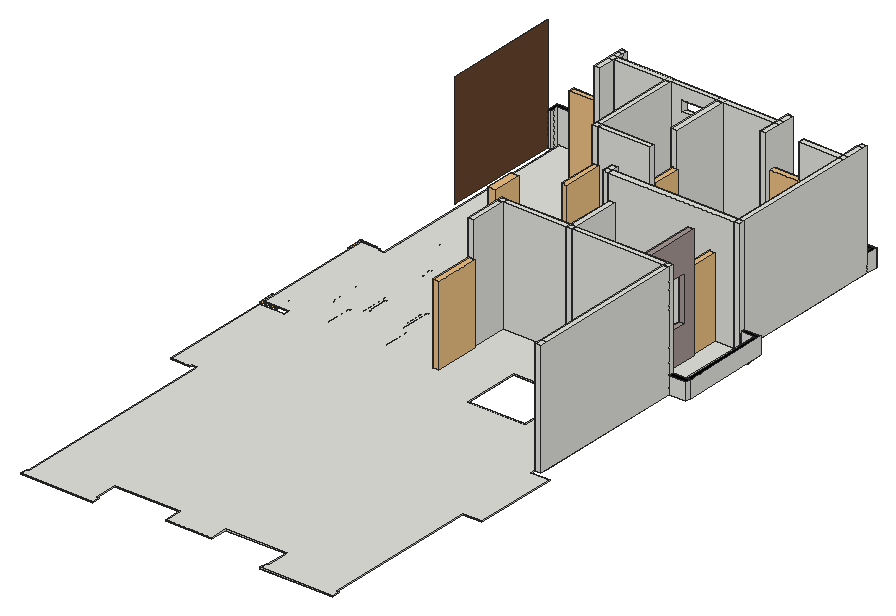
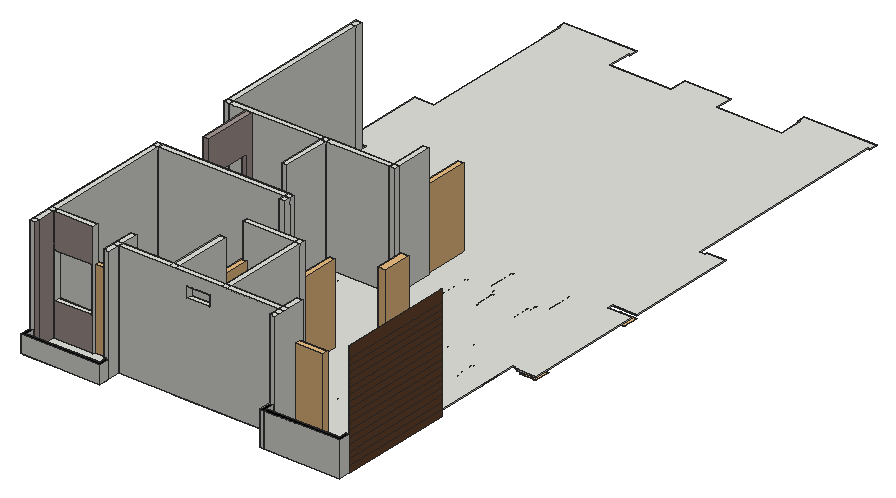
# SketchUp Ruby script. Lengths in inches.
U = 1.inch
M = Sketchup.active_model
def pt(a) = Geom::Point3d.new(a.map { |v| v * U })
def face(e, loops, mat)
  f = e.add_face(loops[0].map { |a| pt(a) })
  loops[1..].each { |l| e.add_face(l.map { |a| pt(a) }).erase! }
  f.material = f.back_material = mat if mat
  f
end
# faces: each face lists its corners as indices into pts; further lists are holes
def faces(e, pts, list, mat = nil) = list.each { |f| face(e, (f[0].is_a?(Array) ? f : [f]).map { |l| l.map { |i| pts[i] } }, mat) }
# xy, xz, yz: faces in a plane at the given z, y or x. An outline is a flat list of corners, or four numbers for a rectangle; further outlines are holes
def ring(l) = l.size == 4 ? [[l[0], l[1]], [l[2], l[1]], [l[2], l[3]], [l[0], l[3]]] : l.each_slice(2).to_a
def flat(e, list, mat, &to3) = list.each { |f| face(e, (f[0].is_a?(Array) ? f : [f]).map { |l| ring(l).map { |u, v| to3.(u, v) } }, mat) }
def xy(e, z, list, mat = nil) = flat(e, list, mat) { |x, y| [x, y, z] }
def xz(e, y, list, mat = nil) = flat(e, list, mat) { |x, z| [x, y, z] }
def yz(e, x, list, mat = nil) = flat(e, list, mat) { |y, z| [x, y, z] }
def lines(e, pts, list) = list.each { |a, b| e.add_line(pt(pts[a]), pt(pts[b])) }
# prism: a flat outline (further loops are holes) pulled along v
def prism(e, loops, v, mat = nil)
  f = face(e, loops, mat); d = Geom::Vector3d.new(v.map { |x| x * U })
  f.pushpull(f.normal.samedirection?(d) ? d.length : -d.length)
end
def box(e, o, s, mat = nil) = prism(e, [[o, [o[0] + s[0], o[1], o[2]], [o[0] + s[0], o[1] + s[1], o[2]], [o[0], o[1] + s[1], o[2]]]], [0, 0, s[2]], mat)
def at(x, y, z, deg = 0) = Geom::Transformation.translation(pt([x, y, z])) * Geom::Transformation.rotation(ORIGIN, Z_AXIS, deg.degrees)
def axes(o, x, y, z) = Geom::Transformation.new([*x, 0, *y, 0, *z, 0, *pt(o).to_a, 1])
def part(name) = M.definitions.add(name)
# library, detail: a bought-in or finely detailed component or shape, given as its bounding box
def library(name, o, s) = part(name).tap { |d| box(d.entities, o, s) }
def detail(e, o, s) = box(e.add_group.entities, o, s)
def put(e, d, t, mat = nil) = e.add_instance(d, t).tap { |i| i.material = mat if mat }
def group(e, t, mat = nil) = e.add_group.tap { |g| g.transformation = t; g.material = mat if mat }.entities
root = M.entities
M.materials.add("M09_Shadow_Night").color = [0, 0, 0]
M.materials.add("Marble_06_1K").color = [165, 150, 147]
M.materials.add("Wood_Veneer_15_1K").color = [103, 69, 45]
c1 = part("Group\#84")
xy(c1.entities,0,[[[-2,-32,-2,-24,0.04,-24,0.04,0,0,0,0,198,-6,198,-6,196,-25.9,196,-25.9,312.57,0,312.57,0,318.21,-25.9,318.21,-25.9,446,-6,446,-6,444,0,444,0,675.78,72,673.93,76,673.93,76,665.93,74,665.93,74,636,252.4,636,252.4,673.93,328.4,673.93,328.4,636,324.4,636,324.4,498.14,330.4,498.14,330.4,499.84,344.35,499.84,344.35,411,324.4,411,324.4,231,344.35,231,344.35,142,324.4,142,324.4,0,324.58,0,324.58,-24,326.4,-24,326.4,-32,250.4,-32,250.4,-24,252.4,-24,252.4,0,188.4,0,188.4,-18,140,-18,140,0,72,0,72,-24,74,-24,74,-32],[210.4,291,270.4,351]]])
xy(c1.entities,1,[[[-2,-32,74,-32,74,-24,72,-24,72,0,140,0,140,-18,188.4,-18,188.4,0,252.4,0,252.4,-24,250.4,-24,250.4,-32,326.4,-32,326.4,-24,324.58,-24,324.58,0,324.4,0,324.4,142,344.35,142,344.35,231,324.4,231,324.4,411,344.35,411,344.35,499.84,330.4,499.84,330.4,498.14,324.4,498.14,324.4,636,328.4,636,328.4,673.93,252.4,673.93,252.4,636,74,636,74,665.93,76,665.93,76,673.93,72,673.93,0,675.78,0,444,-6,444,-6,446,-25.9,446,-25.9,318.21,0,318.21,0,312.57,-25.9,312.57,-25.9,196,-6,196,-6,198,0,198,0,0,0.04,0,0.04,-24,-2,-24],[210.4,291,270.4,351]]])
xz(c1.entities,-32,[[-2,0,74,1],[250.4,0,326.4,1]])
xz(c1.entities,-24,[[-2,0,0.04,1],[72,0,74,1],[250.4,0,252.4,1],[324.58,0,326.4,1]])
xz(c1.entities,-18,[[140,0,188.4,1]])
xz(c1.entities,0,[[0,0,0.04,1],[72,0,140,1],[188.4,0,252.4,1],[324.4,0,324.58,1]])
xz(c1.entities,142,[[324.4,0,344.35,1]])
xz(c1.entities,196,[[-25.9,0,-6,1]])
xz(c1.entities,198,[[-6,0,0,1]])
xz(c1.entities,231,[[324.4,0,344.35,1]])
xz(c1.entities,291,[[210.4,0,270.4,1]])
xz(c1.entities,312.57,[[-25.9,0,0,1]])
xz(c1.entities,318.21,[[-25.9,0,0,1]])
xz(c1.entities,351,[[210.4,0,270.4,1]])
xz(c1.entities,411,[[324.4,0,344.35,1]])
xz(c1.entities,444,[[-6,0,0,1]])
xz(c1.entities,446,[[-25.9,0,-6,1]])
xz(c1.entities,498.14,[[324.4,0,330.4,1]])
xz(c1.entities,499.84,[[330.4,0,344.35,1]])
xz(c1.entities,636,[[74,0,252.4,1],[324.4,0,328.4,1]])
xz(c1.entities,665.93,[[74,0,76,1]])
xz(c1.entities,673.93,[[72,0,76,1],[252.4,0,328.4,1]])
yz(c1.entities,-25.9,[[196,0,312.57,1],[318.21,0,446,1]])
yz(c1.entities,-6,[[196,0,198,1],[444,0,446,1]])
yz(c1.entities,-2,[[-32,0,-24,1]])
yz(c1.entities,0,[[0,0,198,1],[312.57,0,318.21,1],[444,0,636,1],[636,0,637.85,1],[637.85,0,675.78,1]])
yz(c1.entities,0.04,[[-24,0,0,1]])
yz(c1.entities,72,[[-24,0,0,1]])
yz(c1.entities,74,[[-32,0,-24,1],[636,0,665.93,1]])
yz(c1.entities,76,[[665.93,0,673.93,1]])
yz(c1.entities,140,[[-18,0,0,1]])
yz(c1.entities,188.4,[[-18,0,0,1]])
yz(c1.entities,210.4,[[291,0,351,1]])
yz(c1.entities,250.4,[[-32,0,-24,1]])
yz(c1.entities,252.4,[[-24,0,0,1],[636,0,673.93,1]])
yz(c1.entities,270.4,[[291,0,351,1]])
yz(c1.entities,324.4,[[0,0,142,1],[231,0,411,1],[498.14,0,636,1]])
yz(c1.entities,324.58,[[-24,0,0,1]])
yz(c1.entities,326.4,[[-32,0,-24,1]])
yz(c1.entities,328.4,[[636,0,673.93,1]])
yz(c1.entities,330.4,[[498.14,0,499.84,1]])
yz(c1.entities,344.35,[[142,0,231,1],[411,0,499.84,1]])
# 3 loose lines left out
p = [[77.67,648,0],[77.67,636,1],[246.4,636,1],[246.4,648,0],[72,673.93,0],[0,675.78,0],
  [0,675.78,1],[72,673.93,1]]
faces(c1.entities,p,[[0,1,2,3],[4,5,6,7]])
c2 = library("TREE-26",[-60.96,-72.91,0],[121.92,134.74,0.01])
c3 = library("HYHHYHYHYHYHY",[-2.09,-4.54,0],[4.18,9.08,0.01])
c4 = library("Group\#51",[0,0,0],[6.9375,42,86.5])
c5 = part("feeeeeeeeee")
p = [[-2.68,3.51,0],[-2.68,3.16,0],[-2.92,3.16,0],[-2.92,3.07,0],[-3.56,3.07,0],[-3.56,3.51,0],
  [-2.68,-3.51,0],[-2.68,-3.16,0],[-2.92,-3.16,0],[-2.92,-3.07,0],[-3.56,-3.07,0],[-3.56,-3.51,0],
  [3.56,3.16,0],[-2.68,2.93,0],[3.56,2.93,0],[-2.48,-3.13,0],[-2.04,-3.07,0],[-1.61,-2.98,0],
  [-1.1875,-2.86,0],[-0.77,-2.72,0],[-0.36,-2.55,0],[0.03,-2.35,0],[0.41,-2.13,0],[0.78,-1.88,0],
  [1.125,-1.62,0],[1.46,-1.32,0],[1.77,-1.01,0],[2.06,-0.68,0],[2.33,-0.33,0],[2.57,0.03,0],
  [2.79,0.42,0],[2.99,0.81,0],[3.16,1.22,0],[3.3,1.63,0],[3.41,2.06,0],[3.5,2.49,0]]
lines(c5.entities,p,[[0,1],[1,2],[2,3],[3,4],[4,5],[5,0],[6,7],[7,8],[8,9],[9,10],[10,11],[11,6],
  [1,12],[13,14],[1,13],[12,14],[8,15],[15,16],[16,17],[17,18],[18,19],[19,20],[20,21],[21,22],
  [22,23],[23,24],[24,25],[25,26],[26,27],[27,28],[28,29],[29,30],[30,31],[31,32],[32,33],[33,34],
  [34,35],[35,14]])
c6 = part("Group\#12")
xy(c6.entities,0,[[0,0,6,7.18],[0,7.18,6,168],[-174.4,129.21,-168.4,168],[-174.4,168,-168.4,174],[-168.4,168,-102,174],
  [-102,168,-96,174],[-96,168,0,174],[0,168,6,174],[6,168,24,174],[-102,174,-96,225]])
xy(c6.entities,18,[[6,168,24,174]],"M09_Shadow_Night")
xy(c6.entities,120,[[0,0,6,7.18],[0,7.18,6,168],[-174.4,129.21,-168.4,168],[-174.4,168,-168.4,174],[-168.4,168,-102,174],
  [-102,168,-96,174],[-96,168,0,174],[0,168,6,174],[-102,174,-96,225]])
xz(c6.entities,0,[[0,0,6,120]])
xz(c6.entities,129.21,[[-174.4,0,-168.4,120]])
xz(c6.entities,168,[[-174.4,0,-168.4,120],[-168.4,0,-102,120],[-102,0,-96,120],[-96,0,0,120],[0,0,6,120],
  [6,0,24,18]])
xz(c6.entities,174,[[-174.4,0,-168.4,120],[-168.4,0,-102,120],[-102,0,-96,120],[-96,0,0,120],[0,0,6,120],
  [6,0,24,18]])
xz(c6.entities,225,[[-102,0,-96,120]])
yz(c6.entities,-174.4,[[129.21,0,168,120],[168,0,174,120]])
yz(c6.entities,-168.4,[[129.21,0,168,120],[168,0,174,120]])
yz(c6.entities,-102,[[168,0,174,120],[174,0,225,120]])
yz(c6.entities,-96,[[168,0,174,120],[174,0,225,120]])
yz(c6.entities,0,[[0,0,7.18,120],[7.18,0,168,120],[168,0,174,120]])
yz(c6.entities,6,[[0,0,168,120],[168,0,174,18],[168,18,174,120]])
yz(c6.entities,24,[[168,0,174,18]])
c7 = library("VVVV",[-3.39,-3.68,0],[6.78,7.36,0.01])
c8 = library("BFGFV",[-4.32,-2.51,0],[8.64,5.02,0.01])
c9 = library("burner",[-300,-225,0],[600,450,0.01])
c10 = library("lcd-01",[-577.99,-134.75,0],[1155.98,269.5,0.01])
c11 = part("Component\#5")
p = [[1166.02,522.1,0],[1167.27,522.1,0],[1183.11,522.1,0],[1183.72,522.1,0],[1165.72,517.1,0],[1167.27,517.1,0],
  [1183.11,517.1,0],[1183.72,517.1,0],[1165.72,512.1,0],[1167.27,512.1,0],[1183.11,512.1,0],[1183.72,512.1,0],
  [1165.72,507.1,0],[1167.27,507.1,0],[1183.11,507.1,0],[1183.72,507.1,0],[1165.72,502.1,0],[1167.27,502.1,0],
  [1183.11,502.1,0],[1183.72,502.1,0],[1165.72,497.1,0],[1167.27,497.1,0],[1183.11,497.1,0],[1183.72,497.1,0],
  [1165.72,492.1,0],[1183.72,492.1,0],[1165.72,487.1,0],[1183.72,487.1,0],[1111.72,482.1,0],[1128.65,482.1,0],
  [1150.05,482.1,0],[1183.72,482.1,0],[1111.72,477.1,0],[1128.65,477.1,0],[1150.05,477.1,0],[1183.72,477.1,0],
  [1111.72,472.1,0],[1128.65,472.1,0],[1150.05,472.1,0],[1173.72,472.1,0],[1117.28,469.6,0],[1112.28,474.6,0],
  [1127.28,479.6,0],[1122.28,484.6,0],[1157.28,469.6,0],[1152.28,474.6,0],[1173.72,473.16,0],[1172.28,474.6,0],
  [1167.28,479.6,0],[1162.28,484.6,0],[1183.72,483.16,0],[1182.28,484.6,0],[1177.28,489.6,0],[1172.48,494.4,0],
  [1167.27,499.61,0],[1165.72,501.16,0],[1183.72,503.16,0],[1183.11,503.77,0],[1167.27,519.61,0],[1165.77,521.11,0],
  [1183.72,523.16,0],[1182.3,524.58,0],[1118.53,469.6,0],[1113.53,474.6,0],[1128.53,479.6,0],[1123.53,484.6,0],
  [1158.53,469.6,0],[1153.53,474.6,0],[1173.72,474.41,0],[1173.53,474.6,0],[1168.53,479.6,0],[1163.53,484.6,0],
  [1183.72,484.41,0],[1183.53,484.6,0],[1178.53,489.6,0],[1173.73,494.4,0],[1167.27,500.86,0],[1165.72,502.41,0],
  [1183.72,504.41,0],[1183.53,504.6,0],[1167.27,520.86,0],[1166.02,522.11,0],[1183.72,524.41,0],[1183.55,524.58,0],
  [1119.78,469.6,0],[1114.78,474.6,0],[1128.65,480.73,0],[1124.78,484.6,0],[1159.78,469.6,0],[1154.78,474.6,0],
  [1169.78,479.6,0],[1164.78,484.6,0],[1179.78,489.6,0],[1174.98,494.4,0],[1167.27,502.11,0],[1165.72,503.66,0],
  [1167.27,522.11,0],[1166.48,522.9,0]]
lines(c11.entities,p,[[0,1],[2,3],[4,5],[6,7],[8,9],[10,11],[12,13],[14,15],[16,17],[18,19],[20,21],[22,23],
  [24,25],[26,27],[28,29],[30,31],[32,33],[34,35],[36,37],[38,39],[40,41],[42,43],[44,45],[46,47],
  [48,49],[50,51],[52,53],[54,55],[56,57],[58,59],[60,61],[62,63],[64,65],[66,67],[68,69],[70,71],
  [72,73],[74,75],[76,77],[78,79],[80,81],[82,83],[84,85],[86,87],[88,89],[90,91],[92,93],[94,95],
  [96,97]])
c12 = library("sink",[-449.92,-250,0],[899.84,500,0.01])
c13 = library("A$C72E23588",[-1177.7,-903.95,0],[2355.4,1807.9,0.01])
c14 = part("Group\#14")
xy(c14.entities,0,[[0,0,4.05,3.45],[0,3.45,4.05,88.84],[-13.95,88.84,0,93],[0,88.84,4.05,93]])
xy(c14.entities,18,[[0,0,4.05,88.84],[-13.95,88.84,0,93],[0,88.84,4.05,93]],"M09_Shadow_Night")
xz(c14.entities,0,[[0,0,4.05,18]])
xz(c14.entities,88.84,[[-13.95,0,0,18]])
xz(c14.entities,93,[[-13.95,0,4.05,18]])
yz(c14.entities,-13.95,[[88.84,0,93,18]])
yz(c14.entities,0,[[0,0,3.45,18],[3.45,0,88.84,18]])
yz(c14.entities,4.05,[[0,0,93,18]])
c15 = library("JEEW",[-211.14,-299.86,0],[422.28,599.72,0.01])
c16 = library("ghgjg",[-265.23,-341.01,0],[530.46,682.02,0.01])
c17 = part("tgr")
p = [[-2.37,-3.35,0],[-2.37,-2.82,0],[-2.73,-2.82,0],[-2.73,-2.68,0],[-3.71,-2.68,0],[-3.71,-3.35,0],
  [-2.37,3.35,0],[-2.37,2.82,0],[-2.73,2.82,0],[-2.73,2.68,0],[-3.71,2.68,0],[-3.71,3.35,0],
  [3.71,-2.82,0],[-2.37,-2.46,0],[3.71,-2.46,0],[3.7,-2.46,0],[3.63,-2.07,0],[3.53,-1.68,0],
  [3.41,-1.3,0],[3.27,-0.93,0],[3.1,-0.57,0],[2.91,-0.22,0],[2.7,0.12,0],[2.46,0.4375,0],
  [2.21,0.74,0],[1.93,1.03,0],[1.64,1.3,0],[1.33,1.55,0],[1.01,1.79,0],[0.67,1.99,0],
  [0.32,2.18,0],[-0.04,2.35,0],[-0.41,2.49,0],[-0.8,2.6,0],[-1.18,2.69,0],[-1.58,2.76,0],
  [-1.97,2.8,0]]
lines(c17.entities,p,[[0,1],[1,2],[2,3],[3,4],[4,5],[5,0],[6,7],[7,8],[8,9],[9,10],[10,11],[11,6],
  [1,12],[13,14],[1,13],[12,14],[15,16],[16,17],[17,18],[18,19],[19,20],[20,21],[21,22],[22,23],
  [23,24],[24,25],[25,26],[26,27],[27,28],[28,29],[29,30],[30,31],[31,32],[32,33],[33,34],[34,35],
  [35,36],[36,7]])
c18 = library("Group\#49",[0,0,0],[8.31,30,84])
c19 = part("EGWF")
p = [[2.59,-3.49,0],[2.59,-3.09,0],[2.85,-3.09,0],[2.85,-2.99,0],[3.58,-2.99,0],[3.58,-3.49,0],
  [2.59,3.49,0],[2.59,3.09,0],[2.85,3.09,0],[2.85,2.99,0],[3.58,2.99,0],[3.58,3.49,0],
  [-3.58,-3.09,0],[2.59,-2.82,0],[-3.58,-2.82,0],[2.2,3.07,0],[1.81,3.04,0],[1.42,2.97,0],
  [1.03,2.89,0],[0.66,2.78,0],[0.29,2.64,0],[-0.07,2.48,0],[-0.42,2.3,0],[-0.76,2.1,0],
  [-1.08,1.875,0],[-1.39,1.63,0],[-1.68,1.37,0],[-1.96,1.09,0],[-2.21,0.79,0],[-2.45,0.48,0],
  [-2.67,0.15,0],[-2.86,-0.1875,0],[-3.04,-0.54,0],[-3.1875,-0.9,0],[-3.32,-1.28,0],[-3.42,-1.66,0],
  [-3.5,-2.04,0],[-3.55,-2.43,0]]
lines(c19.entities,p,[[0,1],[1,2],[2,3],[3,4],[4,5],[5,0],[6,7],[7,8],[8,9],[9,10],[10,11],[11,6],
  [1,12],[13,14],[1,13],[12,14],[7,15],[15,16],[16,17],[17,18],[18,19],[19,20],[20,21],[21,22],
  [22,23],[23,24],[24,25],[25,26],[26,27],[27,28],[28,29],[29,30],[30,31],[31,32],[32,33],[33,34],
  [34,35],[35,36],[36,37],[37,14]])
c20 = library("double bed",[-999.9375,-1062.5,0],[1999.875,2125,0.01])
c21 = part("Group\#116")
xy(c21.entities,0,[[24,0,24.75,24.75]])
xy(c21.entities,107,[[24,0,24.75,24.75]])
xz(c21.entities,0,[[24,0,24.75,107]])
xz(c21.entities,24.75,[[24,0,24.75,107]])
yz(c21.entities,24,[[0,0,24.75,6],[0,6,24.75,12],[0,12,24.75,18],[0,18,24.75,24],[0,24,24.75,30],
  [0,30,24.75,36],[0,36,24.75,42],[0,42,24.75,48],[0,48,24.75,54],[0,54,24.75,60],
  [0,60,24.75,66],[0,66,24.75,72],[0,72,24.75,78],[0,78,24.75,84],[0,84,24.75,90],
  [0,90,24.75,96],[0,96,24.75,107]],"Wood_Veneer_15_1K")
yz(c21.entities,24.75,[[0,0,24.75,107]])
c22 = part("G5GTGTGT")
p = [[0.52,4.97,0],[0.52,-4.97,0],[0.36,-4.97,0],[0.36,4.97,0],[-0.08,-4.53,0],[-0.08,4.53,0],
  [0.33,4.97,0],[0.3,4.97,0],[0.28,4.96,0],[0.25,4.96,0],[0.22,4.95,0],[0.2,4.94,0],
  [0.17,4.93,0],[0.15,4.92,0],[0.12,4.9,0],[0.1,4.89,0],[0.08,4.87,0],[0.06,4.85,0],
  [0.04,4.83,0],[0.02,4.8125,0],[0,4.79,0],[-0.01,4.77,0],[-0.03,4.74,0],[-0.04,4.72,0],
  [-0.05,4.69,0],[-0.0625,4.67,0],[-0.07,4.64,0],[-0.08,4.61,0],[-0.08,4.59,0],[-0.08,4.56,0],
  [-0.08,-4.56,0],[-0.08,-4.59,0],[-0.08,-4.61,0],[-0.07,-4.64,0],[-0.0625,-4.67,0],[-0.05,-4.69,0],
  [-0.04,-4.72,0],[-0.03,-4.74,0],[-0.01,-4.77,0],[0,-4.79,0],[0.02,-4.8125,0],[0.04,-4.83,0],
  [0.06,-4.85,0],[0.08,-4.87,0],[0.1,-4.89,0],[0.12,-4.9,0],[0.15,-4.92,0],[0.17,-4.93,0],
  [0.2,-4.94,0],[0.22,-4.95,0],[0.25,-4.96,0],[0.28,-4.96,0],[0.3,-4.97,0],[0.33,-4.97,0],
  [-0.08,-1.38,0],[-0.52,-1.38,0],[-0.08,1.38,0],[-0.52,1.38,0]]
lines(c22.entities,p,[[0,1],[1,2],[2,3],[3,0],[4,5],[3,6],[6,7],[7,8],[8,9],[9,10],[10,11],[11,12],
  [12,13],[13,14],[14,15],[15,16],[16,17],[17,18],[18,19],[19,20],[20,21],[21,22],[22,23],[23,24],
  [24,25],[25,26],[26,27],[27,28],[28,29],[29,5],[4,30],[30,31],[31,32],[32,33],[33,34],[34,35],
  [35,36],[36,37],[37,38],[38,39],[39,40],[40,41],[41,42],[42,43],[43,44],[44,45],[45,46],[46,47],
  [47,48],[48,49],[49,50],[50,51],[51,52],[52,53],[53,2],[54,55],[56,57],[55,57]])
c23 = part("Group\#15")
xy(c23.entities,0,[[60,-108.67,66,-102.67],[66,-108.67,120.4,-102.67],[60,-102.67,66,-12.67],[114.4,-72.67,120.4,-12.67],[0,-30.67,6,-12.67],
  [174.4,-30.67,180.4,-12.67],[0,-12.67,6,-6.67],[6,-12.67,60,-6.67],[60,-12.67,66,-6.67],[66,-12.67,114.4,-6.67],
  [114.4,-12.67,120.4,-6.67],[120.4,-12.67,174.4,-6.67],[174.4,-12.67,180.4,-6.67],[0,-6.67,6,0],[174.4,-6.67,180.4,5.26],
  [0,0,6,5.26]])
xy(c23.entities,96,[[78,-12.67,102.4,-6.67]])
xy(c23.entities,108,[[78,-12.67,102.4,-6.67]])
xy(c23.entities,120,[[60,-108.67,66,-102.67],[66,-108.67,120.4,-102.67],[60,-102.67,66,-12.67],[114.4,-72.67,120.4,-12.67],[0,-30.67,6,-12.67],
  [174.4,-30.67,180.4,-12.67],[0,-12.67,6,-6.67],[6,-12.67,60,-6.67],[60,-12.67,66,-6.67],[66,-12.67,114.4,-6.67],
  [114.4,-12.67,120.4,-6.67],[120.4,-12.67,174.4,-6.67],[174.4,-12.67,180.4,-6.67],[0,-6.67,6,0],[174.4,-6.67,180.4,5.26],
  [0,0,6,5.26]])
xz(c23.entities,-108.67,[[60,0,66,120],[66,0,120.4,120]])
xz(c23.entities,-102.67,[[60,0,66,120],[66,0,120.4,120]])
xz(c23.entities,-72.67,[[114.4,0,120.4,120]])
xz(c23.entities,-30.67,[[0,0,6,120],[174.4,0,180.4,120]])
xz(c23.entities,-12.67,[[6,0,60,120],[60,0,66,120],[[66,0,114.4,120],[78,96,102.4,108]],[114.4,0,120.4,120],[120.4,0,174.4,120]])
xz(c23.entities,-6.67,[[[6,0,174.4,120],[78,96,102.4,108]]])
xz(c23.entities,5.26,[[0,0,6,120],[174.4,0,180.4,120]])
yz(c23.entities,0,[[-30.67,0,5.26,120]])
yz(c23.entities,6,[[-30.67,0,-12.67,120],[-12.67,0,-6.67,120],[-6.67,0,0,120],[0,0,5.26,120]])
yz(c23.entities,60,[[-108.67,0,-102.67,120],[-102.67,0,-12.67,120]])
yz(c23.entities,66,[[-108.67,0,-102.67,120],[-102.67,0,-12.67,120]])
yz(c23.entities,78,[[-12.67,96,-6.67,108]])
yz(c23.entities,102.4,[[-12.67,96,-6.67,108]])
yz(c23.entities,114.4,[[-72.67,0,-12.67,120]])
yz(c23.entities,120.4,[[-108.67,0,-102.67,120],[-72.67,0,-12.67,120]])
yz(c23.entities,174.4,[[-30.67,0,-12.67,120],[-12.67,0,-6.67,120],[-6.67,0,5.26,120]])
yz(c23.entities,180.4,[[-30.67,0,5.26,120]])
c24 = library("Group\#48",[0,0,0],[6.9375,42,86.5])
c25 = library("Component\#3",[961.32,686.58,0],[54,18,0.01])
c26 = library("Component\#4",[1075.72,686.58,0],[54,18,0.01])
c27 = part("Group\#16")
xy(c27.entities,0,[[0,0,4,3.74],[80,0,84,8],[0,3.74,4,8],[0,8,4,12],[4,8,80,12],
  [80,8,84,12]])
xy(c27.entities,18,[[0,0,4,12],[80,0,84,0,84,12,4,12,4,8,80,8]],"M09_Shadow_Night")
xz(c27.entities,0,[[0,0,4,18],[80,0,84,18]])
xz(c27.entities,8,[[4,0,80,18]])
xz(c27.entities,12,[[0,0,84,18]])
yz(c27.entities,0,[[0,0,12,18]])
yz(c27.entities,4,[[0,0,3.74,18],[3.74,0,8,18]])
yz(c27.entities,80,[[0,0,8,18]])
yz(c27.entities,84,[[0,0,12,18]])
c28 = part("Group\#13")
xy(c28.entities,0,[[0,0,4,3.01],[80,0,84,8],[0,3.01,4,8],[0,8,4,12],[4,8,80,12],
  [80,8,84,12]])
xy(c28.entities,36,[[0,0,4,12],[80,0,84,12],[4,8,80,12]],"M09_Shadow_Night")
xz(c28.entities,0,[[0,0,4,36],[80,0,84,36]])
xz(c28.entities,8,[[4,0,80,36]])
xz(c28.entities,12,[[0,0,80,36],[80,0,84,36]])
yz(c28.entities,0,[[0,0,12,36]])
yz(c28.entities,4,[[0,0,3.01,36],[3.01,0,8,36]])
yz(c28.entities,80,[[0,0,8,36],[8,0,12,36]])
yz(c28.entities,84,[[0,0,12,36]])
prism(root,[[[338.2,484.34,372],[338.2,541.34,372],[338.2,541.34,492],[338.2,484.34,492]],[[338.2,490.34,408],[338.2,490.34,456],[338.2,529.34,456],[338.2,529.34,408]]],[-6,0,0],"Marble_06_1K")
box(root,[224.2,703.34,372],[54,18,1])
xy(root,372,[[218.2,571.34,362.2,571.34,362.2,739.27,356.2,739.27,356.2,715.34,314.2,715.34,314.2,709.34,356.2,709.34,356.2,577.34,224.2,577.34,224.2,583.34,218.2,583.34]],"Marble_06_1K")
put(root,c1,at(31.8,73.34,372))
put(root,c2,axes([12.58,398.13,372],[0,0.1317,0],[0.1317,0,0],[0,0,0.1317]),"Marble_06_1K")
put(root,c3,axes([99.08,410.24,372],[0,-6.75189,0],[6.75189,0,0],[0,0,6.75189]),"Marble_06_1K")
put(root,c4,axes([189.46,439.01,372],[-0.85622,0,0],[0,-1.13,0],[0,0,0.9711]))
put(root,c5,axes([163.46,415.55,372],[-6.83664,0,0],[0,-6.83664,0],[0,0,6.83664]),"Marble_06_1K")
put(root,c6,at(356.2,310.34,372))
put(root,c7,axes([138,443.33,372],[-4.47564,0,0],[0,4.47564,0],[0,0,4.47564]),"Marble_06_1K")
put(root,c7,axes([64.42,443.33,372],[4.47564,0,0],[0,4.47564,0],[0,0,4.47564]),"Marble_06_1K")
put(root,c8,axes([101.4,444.26,372],[4.3395,0,0],[0,4.3395,0],[0,0,4.3395]),"Marble_06_1K")
put(root,c2,axes([371.8,491.09,372],[0,0.1317,0],[0.1317,0,0],[0,0,0.1317]),"Marble_06_1K")
put(root,c9,axes([287.83,493.58,372],[-0.03566,0,0],[0,-0.03566,0],[0,0,0.03566]),"Marble_06_1K")
put(root,c10,axes([102.68,511.95,372],[0.04,0,0],[0,0.04,0],[0,0,0.04]),"Marble_06_1K")
put(root,c11,at(-851.52,16.76,372),"Marble_06_1K")
put(root,c2,axes([12.58,513.99,372],[0,0.1317,0],[0.1317,0,0],[0,0,0.1317]),"Marble_06_1K")
put(root,c12,axes([323.67,525.41,372],[0,0.03168,0],[0.03168,0,0],[0,0,0.03168]),"Marble_06_1K")
put(root,c13,axes([191.83,525.47,372],[0.0356,0,0],[0,-0.0356,0],[0,0,0.0356]),"Marble_06_1K")
put(root,c14,at(376.15,484.34,372))
put(root,c15,axes([106.95,532.38,372],[0,-0.04284,0],[-0.04284,0,0],[0,0,0.04284]),"Marble_06_1K")
put(root,c16,axes([45.4375,547.34,372],[0,-0.04,0],[-0.04,0,0],[0,0,0.04]),"Marble_06_1K")
put(root,c17,axes([348.8,556.34,372],[4.47464,0,0],[0,-4.47464,0],[0,0,4.47464]),"Marble_06_1K")
put(root,c4,axes([330.54,541.34,372],[0.85622,0,0],[0,0.71429,0],[0,0,0.9711]))
put(root,c17,axes([109.2,556.34,372],[-4.47464,0,0],[0,-4.47464,0],[0,0,4.47464]),"Marble_06_1K")
put(root,c18,at(121.52,541.34,372))
put(root,c2,axes([371.8,567.61,372],[0,0.1317,0],[0.1317,0,0],[0,0,0.1317]),"Marble_06_1K")
put(root,c19,axes([239.8,604.34,372],[-6.02515,0,0],[0,6.02515,0],[0,0,6.02515]),"Marble_06_1K")
put(root,c19,axes([148.2,604.34,372],[6.02515,0,0],[0,6.02515,0],[0,0,6.02515]),"Marble_06_1K")
put(root,c18,axes([222.48,625.34,372],[-1,0,0],[0,-1.4,0],[0,0,1]))
put(root,c4,axes([171.46,625.34,372],[-0.85622,0,0],[0,-1,0],[0,0,0.9711]))
put(root,c20,axes([71.06,633.07,372],[0,-0.03695,0],[-0.03695,0,0],[0,0,0.03695]),"Marble_06_1K")
put(root,c20,axes([316.9375,633.07,372],[0,-0.03695,0],[0.03695,0,0],[0,0,0.03695]),"Marble_06_1K")
put(root,c15,axes([178.84,644.18,372],[-0.04284,0,0],[0,0.04284,0],[0,0,0.04284]),"Marble_06_1K")
put(root,c17,axes([207.6,646.34,372],[-4.47464,0,0],[0,4.47464,0],[0,0,4.47464]),"Marble_06_1K")
put(root,c4,axes([225.86,661.34,372],[-0.85622,0,0],[0,-0.71429,0],[0,0,0.9711]))
put(root,c10,axes([158.41,652,372],[0,-0.04,0],[0.04,0,0],[0,0,0.04]),"Marble_06_1K")
g1 = group(root,at(356.2,733.76,372))
xy(g1,0,[[-138,-162.42,-132,-156.42],[-132,-162.42,0,-156.42],[0,-162.42,6,-156.42],[-138,-156.42,-132,-150.42],[0,-156.42,6,-24.42],
  [-42,-24.42,0,-18.42],[0,-24.42,6,-18.42],[0,-18.42,6,0],[0,0,6,5.51]])
xy(g1,36,[[-40,-24.42,-2,-18.42]])
xy(g1,84,[[-40,-24.42,-2,-18.42]])
xy(g1,120,[[-138,-162.42,-132,-156.42],[-132,-162.42,0,-156.42],[0,-162.42,6,-156.42],[-138,-156.42,-132,-150.42],[0,-156.42,6,-24.42],
  [-42,-24.42,0,-18.42],[0,-24.42,6,-18.42],[0,-18.42,6,0],[0,0,6,5.51]])
xz(g1,-162.42,[[-138,0,-132,120],[-132,0,0,120],[0,0,6,120]])
xz(g1,-156.42,[[-138,0,-132,120],[-132,0,0,120],[0,0,6,120]])
xz(g1,-150.42,[[-138,0,-132,120]])
xz(g1,-24.42,[[[-42,0,0,120],[-40,36,-2,84]]])
xz(g1,-18.42,[[[-42,0,0,120],[-40,36,-2,84]]],"Marble_06_1K")
xz(g1,5.51,[[0,0,6,120]])
yz(g1,-138,[[-162.42,0,-156.42,120],[-156.42,0,-150.42,120]])
yz(g1,-132,[[-162.42,0,-156.42,120],[-156.42,0,-150.42,120]])
yz(g1,-42,[[-24.42,0,-18.42,120]])
yz(g1,-40,[[-24.42,36,-18.42,84]])
yz(g1,-2,[[-24.42,36,-18.42,84]])
yz(g1,0,[[-162.42,0,-156.42,120],[-156.42,0,-24.42,120],[-24.42,0,-18.42,120]])
yz(g1,0,[[-18.42,0,0,120],[0,0,5.51,120]],"Marble_06_1K")
yz(g1,6,[[-162.42,0,-156.42,120],[-156.42,0,5.51,120]])
put(root,c21,axes([1.05,618.07,372],[1,0,0],[0,4.89695,0],[0,0,1.1215]),"Wood_Veneer_15_1K")
put(root,c22,axes([226.1,681.76,372],[3.62,0,0],[0,3.62,0],[0,0,3.62]),"Marble_06_1K")
put(root,c23,at(103.8,734.01,372))
put(root,c16,axes([193.9,707.6,372],[-0.04,0,0],[0,0.04,0],[0,0,0.04]),"Marble_06_1K")
put(root,c4,axes([103.8,707.68,372],[0,0.85622,0],[-0.71429,0,0],[0,0,0.97071]))
put(root,c24,axes([314.2,707.68,372],[0,0.85622,0],[-0.71429,0,0],[0,0,0.97071]))
put(root,c25,at(-851.52,16.76,372),"Marble_06_1K")
put(root,c26,at(-851.52,16.76,372),"Marble_06_1K")
put(root,c17,axes([299.2,725.9375,372],[0,4.47464,0],[4.47464,0,0],[0,0,4.47464]),"Marble_06_1K")
put(root,c17,axes([88.8,725.9375,372],[0,4.47464,0],[-4.47464,0,0],[0,0,4.47464]),"Marble_06_1K")
put(root,c2,axes([38.7,741.86,372],[0,0.1317,0],[0.1317,0,0],[0,0,0.1317]),"Marble_06_1K")
put(root,c2,axes([349.66,741.86,372],[0,0.1317,0],[0.1317,0,0],[0,0,0.1317]),"Marble_06_1K")
put(root,c27,at(278.2,739.27,372))
put(root,c28,at(25.8,739.27,372))
